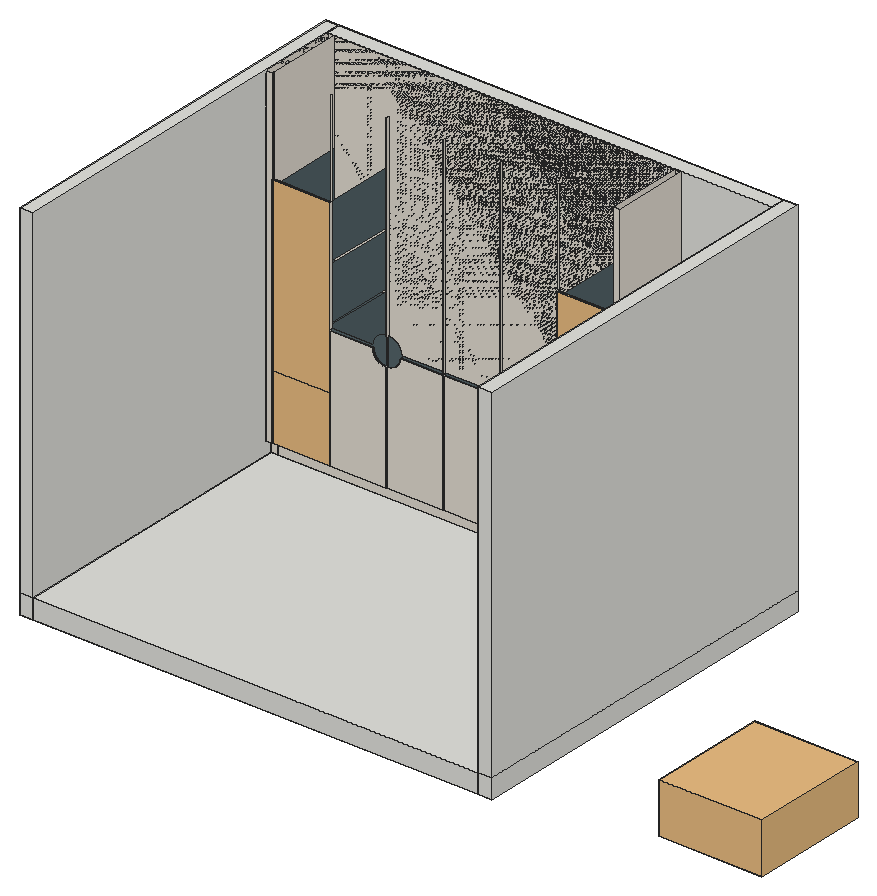
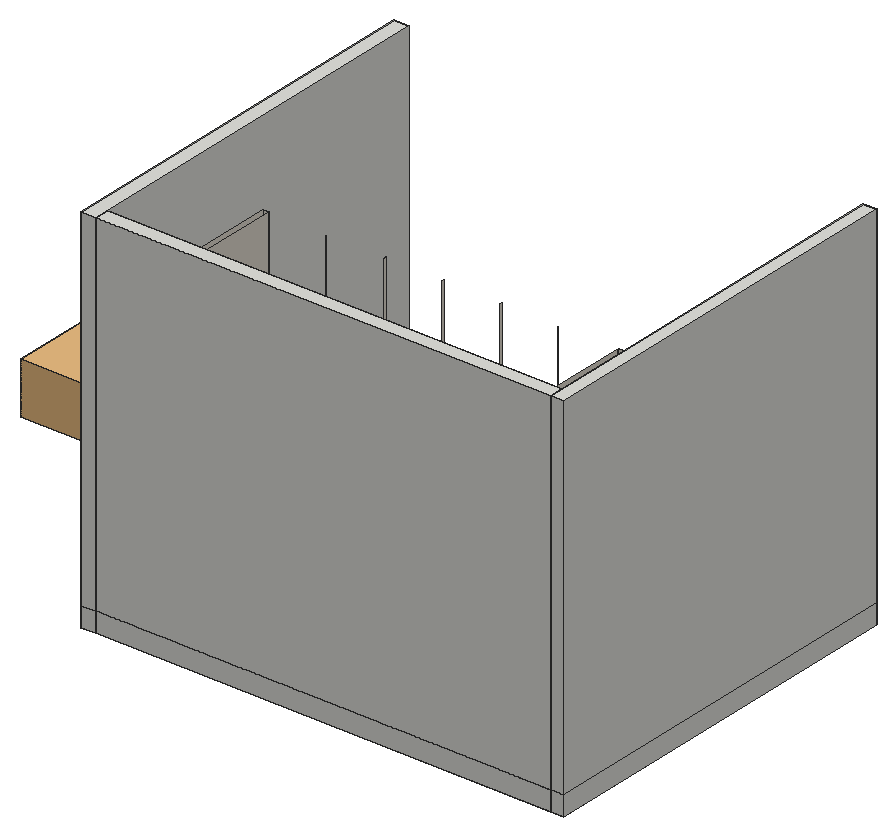
# SketchUp Ruby script. Lengths in millimetres.
U = 1.mm
M = Sketchup.active_model
def pt(a) = Geom::Point3d.new(a.map { |v| v * U })
def face(e, loops, mat)
  f = e.add_face(loops[0].map { |a| pt(a) })
  loops[1..].each { |l| e.add_face(l.map { |a| pt(a) }).erase! }
  f.material = f.back_material = mat if mat
  f
end
# faces: each face lists its corners as indices into pts; further lists are holes
def faces(e, pts, list, mat = nil) = list.each { |f| face(e, (f[0].is_a?(Array) ? f : [f]).map { |l| l.map { |i| pts[i] } }, mat) }
# xy, xz, yz: faces in a plane at the given z, y or x. An outline is a flat list of corners, or four numbers for a rectangle; further outlines are holes
def ring(l) = l.size == 4 ? [[l[0], l[1]], [l[2], l[1]], [l[2], l[3]], [l[0], l[3]]] : l.each_slice(2).to_a
def flat(e, list, mat, &to3) = list.each { |f| face(e, (f[0].is_a?(Array) ? f : [f]).map { |l| ring(l).map { |u, v| to3.(u, v) } }, mat) }
def xy(e, z, list, mat = nil) = flat(e, list, mat) { |x, y| [x, y, z] }
def xz(e, y, list, mat = nil) = flat(e, list, mat) { |x, z| [x, y, z] }
def yz(e, x, list, mat = nil) = flat(e, list, mat) { |y, z| [x, y, z] }
def lines(e, pts, list) = list.each { |a, b| e.add_line(pt(pts[a]), pt(pts[b])) }
# prism: a flat outline (further loops are holes) pulled along v
def prism(e, loops, v, mat = nil)
  f = face(e, loops, mat); d = Geom::Vector3d.new(v.map { |x| x * U })
  f.pushpull(f.normal.samedirection?(d) ? d.length : -d.length)
end
def box(e, o, s, mat = nil) = prism(e, [[o, [o[0] + s[0], o[1], o[2]], [o[0] + s[0], o[1] + s[1], o[2]], [o[0], o[1] + s[1], o[2]]]], [0, 0, s[2]], mat)
def at(x, y, z, deg = 0) = Geom::Transformation.translation(pt([x, y, z])) * Geom::Transformation.rotation(ORIGIN, Z_AXIS, deg.degrees)
def axes(o, x, y, z) = Geom::Transformation.new([*x, 0, *y, 0, *z, 0, *pt(o).to_a, 1])
def part(name) = M.definitions.add(name)
# library, detail: a bought-in or finely detailed component or shape, given as its bounding box
def library(name, o, s) = part(name).tap { |d| box(d.entities, o, s) }
def detail(e, o, s) = box(e.add_group.entities, o, s)
def put(e, d, t, mat = nil) = e.add_instance(d, t).tap { |i| i.material = mat if mat }
def group(e, t, mat = nil) = e.add_group.tap { |g| g.transformation = t; g.material = mat if mat }.entities
root = M.entities
M.materials.add("Olon-Denim-Chic-VT14-1K").color = [84, 100, 105]
M.materials.add("Olon-Fresh-Linen-VT10-1K").color = [226, 220, 209]
M.materials.add("Pionite-a-Panolam-Brand-Tidal-Pool-SB045-4K").color = [68, 97, 103]
c1 = part("Group\#1")
xy(c1.entities,0,[[12.7,0,114.3,3048],[114.3,0,3657.6,3048],[3657.6,0,3771.9,3048]])
xy(c1.entities,152.4,[[12.7,0,114.3,3048],[114.3,0,3657.6,3048],[3657.6,0,3771.9,3048]])
xz(c1.entities,0,[[12.7,0,114.3,152.4],[114.3,0,3657.6,152.4],[3657.6,0,3771.9,152.4]])
xz(c1.entities,3048,[[12.7,0,114.3,152.4],[114.3,0,3657.6,152.4],[3657.6,0,3771.9,152.4]])
yz(c1.entities,12.7,[[0,0,3048,152.4]])
yz(c1.entities,114.3,[[0,0,3048,152.4]])
yz(c1.entities,3657.6,[[0,0,3048,152.4]])
yz(c1.entities,3771.9,[[0,0,3048,152.4]])
xy(root,152.4,[[101.6,2374.9,152.4,2933.7],[152.4,2374.9,2870.2,2933.7],[2870.2,2374.9,2921,2933.7]],"Olon-Fresh-Linen-VT10-1K")
xy(root,254,[[101.6,2324.1,101.6,2374.9,152.4,2374.9,152.4,2342.1,149.4,2342.1,149.4,2324.1],[608.4,2324.1,608.4,2342.1,152.4,2342.1,152.4,2374.9,2870.2,2374.9,2870.2,2342.1,2414.2,2342.1,2414.2,2324.1,1967.3,2324.1,1967.3,2342.1,1964.3,2342.1,1964.3,2324.1,1514.3,2324.1,1514.3,2342.1,1511.3,2342.1,1511.3,2324.1,1061.3,2324.1,1061.3,2342.1,1058.3,2342.1,1058.3,2324.1],[2873.2,2324.1,2873.2,2342.1,2870.2,2342.1,2870.2,2374.9,2921,2374.9,2921,2324.1]],"Olon-Fresh-Linen-VT10-1K")
xy(root,279.4,[[177.8,2342.1,580,2904.1],[2442.6,2342.1,2844.8,2904.1]],"Olon-Denim-Chic-VT14-1K")
xy(root,746.5,[[177.8,2342.1,580,2904.1],[2442.6,2342.1,2844.8,2904.1]],"Olon-Denim-Chic-VT14-1K")
xy(root,797.3,[[177.8,2342.1,580,2904.1]],"Olon-Denim-Chic-VT14-1K")
xy(root,797.3,[[2442.6,2342.1,2844.8,2904.1]],"Pionite-a-Panolam-Brand-Tidal-Pool-SB045-4K")
xy(root,1114.7,[[1054.9,2324.1,1058.3,2333.1],[1061.3,2324.1,1064.8,2333.1],[1960.8,2324.1,1964.3,2333.1],[1967.3,2324.1,1970.7,2333.1]],"Olon-Denim-Chic-VT14-1K")
xy(root,1216.3,[[608.4,2324.1,948.1,2333.1]],"Olon-Denim-Chic-VT14-1K")
xz(root,2324.1,[[101.6,254,149.4,2895.6],[608.4,254,1058.3,254,1058.3,1114.7,1054.9,1114.7,1051.4,1114.9,1047.9,1115.2,1044.5,1115.5,1041,1116,1037.6,1116.6,1034.2,1117.3,1030.8,1118.1,1024.2,1120.1,1020.9,1121.2,1017.6,1122.4,1011.2,1125.2,1008.1,1126.7,1005.1,1128.3,1002,1130.1,999.1,1131.9,996.2,1133.8,993.3,1135.8,990.5,1137.9,987.8,1140,982.6,1144.6,980.1,1147.1,977.7,1149.6,975.4,1152.1,973.1,1154.8,970.9,1157.5,966.9,1163.1,965,1166,963.1,1169,961.4,1172,959.8,1175.1,956.8,1181.3,955.5,1184.5,953.1,1191.1,952.1,1194.4,951.2,1197.8,950.4,1201.1,949.7,1204.5,949.1,1208,948.6,1211.4,948.2,1214.9,948.1,1216.3,608.4,1216.3],[1061.3,254,1511.3,254,1511.3,1216.3,1171.6,1216.3,1171.4,1214.9,1171.1,1211.4,1170.6,1208,1170,1204.5,1169.3,1201.1,1168.5,1197.8,1167.5,1194.4,1166.5,1191.1,1165.4,1187.8,1164.2,1184.5,1162.8,1181.3,1161.4,1178.2,1159.9,1175.1,1158.3,1172,1154.7,1166,1152.8,1163.1,1150.8,1160.3,1148.7,1157.5,1146.6,1154.8,1144.3,1152.1,1142,1149.6,1137,1144.6,1134.5,1142.3,1131.8,1140,1129.1,1137.9,1126.3,1135.8,1123.5,1133.8,1120.6,1131.9,1114.6,1128.3,1111.5,1126.7,1108.4,1125.2,1105.3,1123.8,1102,1122.4,1098.8,1121.2,1095.5,1120.1,1092.2,1119.1,1088.8,1118.1,1085.5,1117.3,1082.1,1116.6,1078.6,1116,1075.2,1115.5,1071.7,1115.2,1068.3,1114.9,1064.8,1114.7,1061.3,1114.7],[1514.3,254,1964.3,254,1964.3,1114.7,1960.8,1114.7,1957.3,1114.9,1953.9,1115.2,1950.4,1115.5,1947,1116,1943.5,1116.6,1940.1,1117.3,1936.8,1118.1,1933.4,1119.1,1930.1,1120.1,1926.8,1121.2,1923.6,1122.4,1920.3,1123.8,1917.2,1125.2,1914.1,1126.7,1911,1128.3,1905,1131.9,1902.1,1133.8,1899.3,1135.8,1896.5,1137.9,1893.8,1140,1891.1,1142.3,1888.6,1144.6,1883.6,1149.6,1881.3,1152.1,1879,1154.8,1876.9,1157.5,1874.8,1160.3,1872.8,1163.1,1870.9,1166,1867.3,1172,1865.7,1175.1,1864.2,1178.2,1862.8,1181.3,1861.4,1184.5,1860.2,1187.8,1859.1,1191.1,1858.1,1194.4,1857.1,1197.8,1856.3,1201.1,1855.6,1204.5,1855,1208,1854.5,1211.4,1854.2,1214.9,1854,1216.3,1514.3,1216.3],[1967.3,254,2414.2,254,2414.2,1216.3,2077.5,1216.3,2077.4,1214.9,2077,1211.4,2076.5,1208,2075.9,1204.5,2075.2,1201.1,2074.4,1197.8,2073.5,1194.4,2072.5,1191.1,2070.1,1184.5,2068.8,1181.3,2065.8,1175.1,2064.2,1172,2062.5,1169,2060.6,1166,2058.7,1163.1,2054.7,1157.5,2052.5,1154.8,2050.2,1152.1,2047.9,1149.6,2045.5,1147.1,2043,1144.6,2037.8,1140,2035.1,1137.9,2032.3,1135.8,2029.4,1133.8,2026.5,1131.9,2023.6,1130.1,2020.5,1128.3,2017.5,1126.7,2014.4,1125.2,2008,1122.4,2004.7,1121.2,2001.4,1120.1,1994.8,1118.1,1991.4,1117.3,1988,1116.6,1984.6,1116,1981.1,1115.5,1977.7,1115.2,1974.2,1114.9,1970.7,1114.7,1967.3,1114.7],
  [2873.2,254,2921,2895.6]],"Olon-Fresh-Linen-VT10-1K")
xz(root,2333.1,[[1054.9,1114.7,1058.3,1114.7,1058.3,1335.9,1054.9,1335.8,1047.9,1335.4,1044.5,1335,1041,1334.5,1037.6,1333.9,1034.2,1333.2,1030.8,1332.4,1027.5,1331.5,1020.9,1329.3,1017.6,1328.1,1014.4,1326.8,1011.2,1325.3,1008.1,1323.8,1005.1,1322.2,1002,1320.5,996.2,1316.7,993.3,1314.7,990.5,1312.7,987.8,1310.5,982.6,1305.9,980.1,1303.5,977.7,1301,973.1,1295.8,970.9,1293.1,968.9,1290.3,966.9,1287.4,963.1,1281.6,961.4,1278.5,959.8,1275.5,958.3,1272.4,956.8,1269.2,955.5,1266,953.1,1259.4,952.1,1256.1,951.2,1252.8,950.4,1249.4,949.7,1246,949.1,1242.6,948.6,1239.1,948.2,1235.7,948.1,1234.3,608.4,1234.3,608.4,1216.3,948.1,1216.3,948.2,1214.9,948.6,1211.4,949.1,1208,949.7,1204.5,950.4,1201.1,951.2,1197.8,952.1,1194.4,953.1,1191.1,955.5,1184.5,956.8,1181.3,959.8,1175.1,961.4,1172,963.1,1169,965,1166,966.9,1163.1,970.9,1157.5,973.1,1154.8,975.4,1152.1,977.7,1149.6,980.1,1147.1,982.6,1144.6,987.8,1140,990.5,1137.9,993.3,1135.8,996.2,1133.8,999.1,1131.9,1002,1130.1,1005.1,1128.3,1008.1,1126.7,1011.2,1125.2,1017.6,1122.4,1020.9,1121.2,1024.2,1120.1,1030.8,1118.1,1034.2,1117.3,1037.6,1116.6,1041,1116,1044.5,1115.5,1047.9,1115.2,1051.4,1114.9],[1061.3,1114.7,1064.8,1114.7,1068.3,1114.9,1071.7,1115.2,1075.2,1115.5,1078.6,1116,1082.1,1116.6,1085.5,1117.3,1088.8,1118.1,1092.2,1119.1,1095.5,1120.1,1098.8,1121.2,1102,1122.4,1105.3,1123.8,1108.4,1125.2,1111.5,1126.7,1114.6,1128.3,1120.6,1131.9,1123.5,1133.8,1126.3,1135.8,1129.1,1137.9,1131.8,1140,1134.5,1142.3,1137,1144.6,1142,1149.6,1144.3,1152.1,1146.6,1154.8,1148.7,1157.5,1150.8,1160.3,1152.8,1163.1,1154.7,1166,1158.3,1172,1159.9,1175.1,1161.4,1178.2,1162.8,1181.3,1164.2,1184.5,1165.4,1187.8,1166.5,1191.1,1167.5,1194.4,1168.5,1197.8,1169.3,1201.1,1170,1204.5,1170.6,1208,1171.1,1211.4,1171.4,1214.9,1171.6,1216.3,1511.3,1216.3,1511.3,1234.3,1171.6,1234.3,1171.4,1235.7,1171.1,1239.1,1170.6,1242.6,1170,1246,1169.3,1249.4,1168.5,1252.8,1166.5,1259.4,1165.4,1262.7,1164.2,1266,1161.4,1272.4,1159.9,1275.5,1158.3,1278.5,1156.5,1281.6,1154.7,1284.5,1152.8,1287.4,1150.8,1290.3,1148.7,1293.1,1146.6,1295.8,1142,1301,1139.5,1303.5,1137,1305.9,1134.5,1308.2,1131.8,1310.5,1129.1,1312.7,1123.5,1316.7,1120.6,1318.6,1117.6,1320.5,1114.6,1322.2,1111.5,1323.8,1105.3,1326.8,1102,1328.1,1098.8,1329.3,1092.2,1331.5,1088.8,1332.4,1085.5,1333.2,1082.1,1333.9,1078.6,1334.5,1075.2,1335,1071.7,1335.4,1068.3,1335.6,1064.8,1335.8,1061.3,1335.9],[1960.8,1114.7,1964.3,1114.7,1964.3,1335.9,1960.8,1335.8,1957.3,1335.6,1953.9,1335.4,1950.4,1335,1947,1334.5,1943.5,1333.9,1940.1,1333.2,1936.8,1332.4,1933.4,1331.5,1926.8,1329.3,1923.6,1328.1,1920.3,1326.8,1914.1,1323.8,1911,1322.2,1908,1320.5,1905,1318.6,1902.1,1316.7,1896.5,1312.7,1893.8,1310.5,1891.1,1308.2,1888.6,1305.9,1886.1,1303.5,1883.6,1301,1879,1295.8,1876.9,1293.1,1874.8,1290.3,1872.8,1287.4,1870.9,1284.5,1869.1,1281.6,1867.3,1278.5,1865.7,1275.5,1864.2,1272.4,1861.4,1266,1860.2,1262.7,1859.1,1259.4,1857.1,1252.8,1856.3,1249.4,1855.6,1246,1855,1242.6,1854.5,1239.1,1854.2,1235.7,1854,1234.3,1514.3,1234.3,1514.3,1216.3,1854,1216.3,1854.2,1214.9,1854.5,1211.4,1855,1208,1855.6,1204.5,1856.3,1201.1,1857.1,1197.8,1858.1,1194.4,1859.1,1191.1,1860.2,1187.8,1861.4,1184.5,1862.8,1181.3,1864.2,1178.2,1865.7,1175.1,1867.3,1172,1870.9,1166,1872.8,1163.1,1874.8,1160.3,1876.9,1157.5,1879,1154.8,1881.3,1152.1,1883.6,1149.6,1888.6,1144.6,1891.1,1142.3,1893.8,1140,1896.5,1137.9,1899.3,1135.8,1902.1,1133.8,1905,1131.9,1911,1128.3,1914.1,1126.7,1917.2,1125.2,1920.3,1123.8,1923.6,1122.4,1926.8,1121.2,1930.1,1120.1,1933.4,1119.1,1936.8,1118.1,1940.1,1117.3,1943.5,1116.6,1947,1116,1950.4,1115.5,1953.9,1115.2,1957.3,1114.9],[1967.3,1114.7,1970.7,1114.7,1974.2,1114.9,1977.7,1115.2,1981.1,1115.5,1984.6,1116,1988,1116.6,1991.4,1117.3,1994.8,1118.1,2001.4,1120.1,2004.7,1121.2,2008,1122.4,2014.4,1125.2,2017.5,1126.7,2020.5,1128.3,2023.6,1130.1,2026.5,1131.9,2029.4,1133.8,2032.3,1135.8,2035.1,1137.9,2037.8,1140,2043,1144.6,2045.5,1147.1,2047.9,1149.6,2050.2,1152.1,2052.5,1154.8,2054.7,1157.5,2058.7,1163.1,2060.6,1166,2062.5,1169,2064.2,1172,2065.8,1175.1,2068.8,1181.3,2070.1,1184.5,2072.5,1191.1,2073.5,1194.4,2074.4,1197.8,2075.2,1201.1,2075.9,1204.5,2076.5,1208,2077,1211.4,2077.4,1214.9,2077.5,1216.3,2414.2,1216.3,2414.2,1234.3,2077.5,1234.3,2077.4,1235.7,2077,1239.1,2076.5,1242.6,2075.9,1246,2075.2,1249.4,2074.4,1252.8,2073.5,1256.1,2072.5,1259.4,2070.1,1266,2068.8,1269.2,2067.3,1272.4,2065.8,1275.5,2064.2,1278.5,2062.5,1281.6,2058.7,1287.4,2056.7,1290.3,2054.7,1293.1,2052.5,1295.8,2047.9,1301,2045.5,1303.5,2043,1305.9,2037.8,1310.5,2035.1,1312.7,2032.3,1314.7,2029.4,1316.7,2023.6,1320.5,2020.5,1322.2,2017.5,1323.8,2014.4,1325.3,2011.2,1326.8,2008,1328.1,2004.7,1329.3,1998.1,1331.5,1994.8,1332.4,1991.4,1333.2,1988,1333.9,1984.6,1334.5,1981.1,1335,1977.7,1335.4,1970.7,1335.8,1967.3,1335.9]],"Olon-Denim-Chic-VT14-1K")
xz(root,2342.1,[[149.4,254,152.4,2895.6],[[152.4,254,605.4,770.4],[177.8,279.4,580,746.5]],[605.4,254,608.4,2895.6],[1058.3,254,1061.3,2895.6],[1511.3,254,1514.3,2895.6],
  [1964.3,254,1967.3,2895.6],[2414.2,254,2417.2,2895.6],[[2417.2,254,2870.2,770.4],[2442.6,279.4,2844.8,746.5]],[2870.2,254,2873.2,2895.6],[152.4,770.4,605.4,773.4],
  [2417.2,770.4,2870.2,773.4],[[152.4,773.4,605.4,2132.1],[177.8,797.3,580,2108.2]],[[2417.2,773.4,2870.2,2132.1],[2442.6,797.3,2844.8,2108.2]]],"Olon-Fresh-Linen-VT10-1K")
xz(root,2374.9,[[101.6,152.4,152.4,254],[152.4,152.4,2870.2,254],[2870.2,152.4,2921,254]],"Olon-Fresh-Linen-VT10-1K")
xz(root,2904.1,[[177.8,279.4,580,746.5],[2442.6,279.4,2844.8,746.5],[177.8,797.3,580,1225.3],[2442.6,797.3,2844.8,1225.3]],"Olon-Denim-Chic-VT14-1K")
xz(root,2933.7,[[101.6,152.4,152.4,2895.6],[152.4,152.4,2870.2,2895.6],[2870.2,152.4,2921,2895.6]],"Olon-Fresh-Linen-VT10-1K")
yz(root,101.6,[[2374.9,152.4,2374.9,254,2324.1,254,2324.1,2895.6,2933.7,2895.6,2933.7,152.4]],"Olon-Fresh-Linen-VT10-1K")
yz(root,149.4,[[2324.1,254,2342.1,770.4],[2324.1,770.4,2342.1,773.4],[2324.1,773.4,2342.1,2132.1]],"Olon-Fresh-Linen-VT10-1K")
yz(root,152.4,[[2374.9,152.4,2933.7,152.4,2933.7,2895.6,2342.1,2895.6,2342.1,254,2374.9,254]],"Olon-Fresh-Linen-VT10-1K")
yz(root,177.8,[[2342.1,279.4,2904.1,746.5],[2342.1,797.3,2904.1,797.3,2904.1,1225.3,2344.1,1225.3,2344.1,1243.3,2904.1,1243.3,2904.1,1662.2,2344.1,1662.2,2344.1,1680.2,2904.1,1680.2,2904.1,2108.2,2342.1,2108.2]],"Olon-Denim-Chic-VT14-1K")
yz(root,580,[[2342.1,279.4,2904.1,746.5],[2342.1,797.3,2342.1,2108.2,2904.1,2108.2,2904.1,1680.2,2344.1,1680.2,2344.1,1662.2,2904.1,1662.2,2904.1,1243.3,2344.1,1243.3,2344.1,1225.3,2904.1,1225.3,2904.1,797.3]],"Olon-Denim-Chic-VT14-1K")
yz(root,608.4,[[2324.1,254,2342.1,770.4],[2324.1,770.4,2342.1,773.4],[2324.1,773.4,2324.1,1216.3,2333.1,1216.3,2333.1,1234.3,2324.1,1234.3,2324.1,2132.1,2342.1,2132.1,2342.1,773.4]],"Olon-Fresh-Linen-VT10-1K")
yz(root,1058.3,[[2324.1,254,2342.1,254,2342.1,2895.6,2324.1,2895.6,2324.1,1335.9,2333.1,1335.9,2333.1,1114.7,2324.1,1114.7]],"Olon-Fresh-Linen-VT10-1K")
yz(root,1061.3,[[2324.1,254,2324.1,1114.7,2333.1,1114.7,2333.1,1335.9,2324.1,1335.9,2324.1,2895.6,2342.1,2895.6,2342.1,254]],"Olon-Fresh-Linen-VT10-1K")
yz(root,1511.3,[[2324.1,254,2342.1,254,2342.1,2895.6,2324.1,2895.6,2324.1,1234.3,2333.1,1234.3,2333.1,1216.3,2324.1,1216.3]],"Olon-Fresh-Linen-VT10-1K")
yz(root,1514.3,[[2324.1,254,2324.1,1216.3,2333.1,1216.3,2333.1,1234.3,2324.1,1234.3,2324.1,2895.6,2342.1,2895.6,2342.1,254]],"Olon-Fresh-Linen-VT10-1K")
yz(root,1964.3,[[2324.1,254,2342.1,254,2342.1,2895.6,2324.1,2895.6,2324.1,1335.9,2333.1,1335.9,2333.1,1114.7,2324.1,1114.7]],"Olon-Fresh-Linen-VT10-1K")
yz(root,1967.3,[[2324.1,254,2324.1,1114.7,2333.1,1114.7,2333.1,1335.9,2324.1,1335.9,2324.1,2895.6,2342.1,2895.6,2342.1,254]],"Olon-Fresh-Linen-VT10-1K")
yz(root,2414.2,[[2324.1,254,2342.1,771.9],[2324.1,771.9,2342.1,771.9,2342.1,2133.6,2324.1,2133.6,2324.1,1234.3,2333.1,1234.3,2333.1,1216.3,2324.1,1216.3]],"Olon-Fresh-Linen-VT10-1K")
yz(root,2442.6,[[2342.1,279.4,2904.1,746.5],[2342.1,797.3,2904.1,797.3,2904.1,1225.3,2362.1,1225.3,2362.1,1243.3,2904.1,1243.3,2904.1,1662.2,2362.1,1662.2,2362.1,1680.2,2904.1,1680.2,2904.1,2108.2,2342.1,2108.2]],"Olon-Denim-Chic-VT14-1K")
yz(root,2844.8,[[2342.1,279.4,2904.1,746.5],[2342.1,797.3,2904.1,1225.3]],"Olon-Denim-Chic-VT14-1K")
yz(root,2870.2,[[2374.9,152.4,2374.9,254,2342.1,254,2342.1,2895.6,2933.7,2895.6,2933.7,152.4]],"Olon-Fresh-Linen-VT10-1K")
yz(root,2873.2,[[2324.1,254,2342.1,771.9],[2324.1,771.9,2342.1,2133.6]],"Olon-Fresh-Linen-VT10-1K")
yz(root,2921,[[2374.9,152.4,2933.7,152.4,2933.7,2895.6,2324.1,2895.6,2324.1,254,2374.9,254]],"Olon-Fresh-Linen-VT10-1K")
p = [[1051.4,2324.1,1114.9],[1054.9,2324.1,1114.7],[1054.9,2333.1,1114.7],[1051.4,2333.1,1114.9],[1064.8,2324.1,1114.7],[1068.3,2324.1,1114.9],
  [1068.3,2333.1,1114.9],[1064.8,2333.1,1114.7],[1957.3,2324.1,1114.9],[1960.8,2324.1,1114.7],[1960.8,2333.1,1114.7],[1957.3,2333.1,1114.9],
  [1970.7,2324.1,1114.7],[1974.2,2324.1,1114.9],[1974.2,2333.1,1114.9],[1970.7,2333.1,1114.7],[1047.9,2324.1,1115.2],[1047.9,2333.1,1115.2],
  [1071.7,2324.1,1115.2],[1071.7,2333.1,1115.2],[1953.9,2324.1,1115.2],[1953.9,2333.1,1115.2],[1977.7,2324.1,1115.2],[1977.7,2333.1,1115.2],
  [1044.5,2324.1,1115.5],[1044.5,2333.1,1115.5],[1075.2,2324.1,1115.5],[1075.2,2333.1,1115.5],[1950.4,2324.1,1115.5],[1950.4,2333.1,1115.5],
  [1981.1,2324.1,1115.5],[1981.1,2333.1,1115.5],[1041,2324.1,1116],[1041,2333.1,1116],[1078.6,2324.1,1116],[1078.6,2333.1,1116],
  [1947,2324.1,1116],[1947,2333.1,1116],[1984.6,2324.1,1116],[1984.6,2333.1,1116],[1037.6,2324.1,1116.6],[1037.6,2333.1,1116.6],
  [1082.1,2324.1,1116.6],[1082.1,2333.1,1116.6],[1943.5,2324.1,1116.6],[1943.5,2333.1,1116.6],[1988,2324.1,1116.6],[1988,2333.1,1116.6],
  [1034.2,2324.1,1117.3],[1034.2,2333.1,1117.3],[1085.5,2324.1,1117.3],[1085.5,2333.1,1117.3],[1940.1,2324.1,1117.3],[1940.1,2333.1,1117.3],
  [1991.4,2324.1,1117.3],[1991.4,2333.1,1117.3],[1030.8,2324.1,1118.1],[1030.8,2333.1,1118.1],[1088.8,2324.1,1118.1],[1088.8,2333.1,1118.1],
  [1936.8,2324.1,1118.1],[1936.8,2333.1,1118.1],[1994.8,2324.1,1118.1],[1994.8,2333.1,1118.1],[1027.5,2324.1,1119.1],[1027.5,2333.1,1119.1],
  [1092.2,2324.1,1119.1],[1092.2,2333.1,1119.1],[1933.4,2324.1,1119.1],[1933.4,2333.1,1119.1],[1998.1,2324.1,1119.1],[1998.1,2333.1,1119.1],
  [1024.2,2324.1,1120.1],[1024.2,2333.1,1120.1],[1095.5,2324.1,1120.1],[1095.5,2333.1,1120.1],[1930.1,2324.1,1120.1],[1930.1,2333.1,1120.1],
  [2001.4,2324.1,1120.1],[2001.4,2333.1,1120.1],[1020.9,2324.1,1121.2],[1020.9,2333.1,1121.2],[1098.8,2324.1,1121.2],[1098.8,2333.1,1121.2],
  [1926.8,2324.1,1121.2],[1926.8,2333.1,1121.2],[2004.7,2324.1,1121.2],[2004.7,2333.1,1121.2],[1017.6,2324.1,1122.4],[1017.6,2333.1,1122.4],
  [1102,2324.1,1122.4],[1102,2333.1,1122.4],[1923.6,2324.1,1122.4],[1923.6,2333.1,1122.4],[2008,2324.1,1122.4],[2008,2333.1,1122.4],
  [1014.4,2324.1,1123.8],[1014.4,2333.1,1123.8],[1105.3,2324.1,1123.8],[1105.3,2333.1,1123.8],[1920.3,2324.1,1123.8],[1920.3,2333.1,1123.8],
  [2011.2,2324.1,1123.8],[2011.2,2333.1,1123.8],[1011.2,2324.1,1125.2],[1011.2,2333.1,1125.2],[1108.4,2324.1,1125.2],[1108.4,2333.1,1125.2],
  [1917.2,2324.1,1125.2],[1917.2,2333.1,1125.2],[2014.4,2324.1,1125.2],[2014.4,2333.1,1125.2],[1008.1,2324.1,1126.7],[1008.1,2333.1,1126.7],
  [1111.5,2324.1,1126.7],[1111.5,2333.1,1126.7],[1914.1,2324.1,1126.7],[1914.1,2333.1,1126.7],[2017.5,2324.1,1126.7],[2017.5,2333.1,1126.7],
  [1005.1,2324.1,1128.3],[1005.1,2333.1,1128.3],[1114.6,2324.1,1128.3],[1114.6,2333.1,1128.3],[1911,2324.1,1128.3],[1911,2333.1,1128.3],
  [2020.5,2324.1,1128.3],[2020.5,2333.1,1128.3],[1002,2324.1,1130.1],[1002,2333.1,1130.1],[1117.6,2324.1,1130.1],[1117.6,2333.1,1130.1],
  [1908,2324.1,1130.1],[1908,2333.1,1130.1],[2023.6,2324.1,1130.1],[2023.6,2333.1,1130.1],[999.1,2324.1,1131.9],[999.1,2333.1,1131.9],
  [1120.6,2324.1,1131.9],[1120.6,2333.1,1131.9],[1905,2324.1,1131.9],[1905,2333.1,1131.9],[2026.5,2324.1,1131.9],[2026.5,2333.1,1131.9],
  [996.2,2324.1,1133.8],[996.2,2333.1,1133.8],[1123.5,2324.1,1133.8],[1123.5,2333.1,1133.8],[1902.1,2324.1,1133.8],[1902.1,2333.1,1133.8],
  [2029.4,2324.1,1133.8],[2029.4,2333.1,1133.8],[993.3,2324.1,1135.8],[993.3,2333.1,1135.8],[1126.3,2324.1,1135.8],[1126.3,2333.1,1135.8],
  [1899.3,2324.1,1135.8],[1899.3,2333.1,1135.8],[2032.3,2324.1,1135.8],[2032.3,2333.1,1135.8],[990.5,2324.1,1137.9],[990.5,2333.1,1137.9],
  [1129.1,2324.1,1137.9],[1129.1,2333.1,1137.9],[1896.5,2324.1,1137.9],[1896.5,2333.1,1137.9],[2035.1,2324.1,1137.9],[2035.1,2333.1,1137.9],
  [987.8,2324.1,1140],[987.8,2333.1,1140],[1131.8,2324.1,1140],[1131.8,2333.1,1140],[1893.8,2324.1,1140],[1893.8,2333.1,1140],
  [2037.8,2324.1,1140],[2037.8,2333.1,1140],[985.2,2324.1,1142.3],[985.2,2333.1,1142.3],[1134.5,2324.1,1142.3],[1134.5,2333.1,1142.3],
  [1891.1,2324.1,1142.3],[1891.1,2333.1,1142.3],[2040.4,2324.1,1142.3],[2040.4,2333.1,1142.3],[982.6,2324.1,1144.6],[982.6,2333.1,1144.6],
  [1137,2324.1,1144.6],[1137,2333.1,1144.6],[1888.6,2324.1,1144.6],[1888.6,2333.1,1144.6],[2043,2324.1,1144.6],[2043,2333.1,1144.6],
  [980.1,2324.1,1147.1],[980.1,2333.1,1147.1],[1139.5,2324.1,1147.1],[1139.5,2333.1,1147.1],[1886.1,2324.1,1147.1],[1886.1,2333.1,1147.1],
  [2045.5,2324.1,1147.1],[2045.5,2333.1,1147.1],[977.7,2324.1,1149.6],[977.7,2333.1,1149.6],[1142,2324.1,1149.6],[1142,2333.1,1149.6],
  [1883.6,2324.1,1149.6],[1883.6,2333.1,1149.6],[2047.9,2324.1,1149.6],[2047.9,2333.1,1149.6],[975.4,2324.1,1152.1],[975.4,2333.1,1152.1],
  [1144.3,2324.1,1152.1],[1144.3,2333.1,1152.1],[1881.3,2324.1,1152.1],[1881.3,2333.1,1152.1],[2050.2,2324.1,1152.1],[2050.2,2333.1,1152.1],
  [973.1,2324.1,1154.8],[973.1,2333.1,1154.8],[1146.6,2324.1,1154.8],[1146.6,2333.1,1154.8],[1879,2324.1,1154.8],[1879,2333.1,1154.8],
  [2052.5,2324.1,1154.8],[2052.5,2333.1,1154.8],[970.9,2324.1,1157.5],[970.9,2333.1,1157.5],[1148.7,2324.1,1157.5],[1148.7,2333.1,1157.5],
  [1876.9,2324.1,1157.5],[1876.9,2333.1,1157.5],[2054.7,2324.1,1157.5],[2054.7,2333.1,1157.5],[968.9,2324.1,1160.3],[968.9,2333.1,1160.3],
  [1150.8,2324.1,1160.3],[1150.8,2333.1,1160.3],[1874.8,2324.1,1160.3],[1874.8,2333.1,1160.3],[2056.7,2324.1,1160.3],[2056.7,2333.1,1160.3],
  [966.9,2324.1,1163.1],[966.9,2333.1,1163.1],[1152.8,2324.1,1163.1],[1152.8,2333.1,1163.1],[1872.8,2324.1,1163.1],[1872.8,2333.1,1163.1],
  [2058.7,2324.1,1163.1],[2058.7,2333.1,1163.1],[965,2324.1,1166],[965,2333.1,1166],[1154.7,2324.1,1166],[1154.7,2333.1,1166],
  [1870.9,2324.1,1166],[1870.9,2333.1,1166],[2060.6,2324.1,1166],[2060.6,2333.1,1166],[963.1,2324.1,1169],[963.1,2333.1,1169],
  [1156.5,2324.1,1169],[1156.5,2333.1,1169],[1869.1,2324.1,1169],[1869.1,2333.1,1169],[2062.5,2324.1,1169],[2062.5,2333.1,1169],
  [961.4,2324.1,1172],[961.4,2333.1,1172],[1158.3,2324.1,1172],[1158.3,2333.1,1172],[1867.3,2324.1,1172],[1867.3,2333.1,1172],
  [2064.2,2324.1,1172],[2064.2,2333.1,1172],[959.8,2324.1,1175.1],[959.8,2333.1,1175.1],[1159.9,2324.1,1175.1],[1159.9,2333.1,1175.1],
  [1865.7,2324.1,1175.1],[1865.7,2333.1,1175.1],[2065.8,2324.1,1175.1],[2065.8,2333.1,1175.1],[958.3,2324.1,1178.2],[958.3,2333.1,1178.2],
  [1161.4,2324.1,1178.2],[1161.4,2333.1,1178.2],[1864.2,2324.1,1178.2],[1864.2,2333.1,1178.2],[2067.3,2324.1,1178.2],[2067.3,2333.1,1178.2],
  [956.8,2324.1,1181.3],[956.8,2333.1,1181.3],[1162.8,2324.1,1181.3],[1162.8,2333.1,1181.3],[1862.8,2324.1,1181.3],[1862.8,2333.1,1181.3],
  [2068.8,2324.1,1181.3],[2068.8,2333.1,1181.3],[955.5,2324.1,1184.5],[955.5,2333.1,1184.5],[1164.2,2324.1,1184.5],[1164.2,2333.1,1184.5],
  [1861.4,2324.1,1184.5],[1861.4,2333.1,1184.5],[2070.1,2324.1,1184.5],[2070.1,2333.1,1184.5],[954.3,2324.1,1187.8],[954.3,2333.1,1187.8],
  [1165.4,2324.1,1187.8],[1165.4,2333.1,1187.8],[1860.2,2324.1,1187.8],[1860.2,2333.1,1187.8],[2071.3,2324.1,1187.8],[2071.3,2333.1,1187.8],
  [953.1,2324.1,1191.1],[953.1,2333.1,1191.1],[1166.5,2324.1,1191.1],[1166.5,2333.1,1191.1],[1859.1,2324.1,1191.1],[1859.1,2333.1,1191.1],
  [2072.5,2324.1,1191.1],[2072.5,2333.1,1191.1],[952.1,2324.1,1194.4],[952.1,2333.1,1194.4],[1167.5,2324.1,1194.4],[1167.5,2333.1,1194.4],
  [1858.1,2324.1,1194.4],[1858.1,2333.1,1194.4],[2073.5,2324.1,1194.4],[2073.5,2333.1,1194.4],[951.2,2324.1,1197.8],[951.2,2333.1,1197.8],
  [1168.5,2324.1,1197.8],[1168.5,2333.1,1197.8],[1857.1,2324.1,1197.8],[1857.1,2333.1,1197.8],[2074.4,2324.1,1197.8],[2074.4,2333.1,1197.8],
  [950.4,2324.1,1201.1],[950.4,2333.1,1201.1],[1169.3,2324.1,1201.1],[1169.3,2333.1,1201.1],[1856.3,2324.1,1201.1],[1856.3,2333.1,1201.1],
  [2075.2,2324.1,1201.1],[2075.2,2333.1,1201.1],[949.7,2324.1,1204.5],[949.7,2333.1,1204.5],[1170,2324.1,1204.5],[1170,2333.1,1204.5],
  [1855.6,2324.1,1204.5],[1855.6,2333.1,1204.5],[2075.9,2324.1,1204.5],[2075.9,2333.1,1204.5],[949.1,2324.1,1208],[949.1,2333.1,1208],
  [1170.6,2324.1,1208],[1170.6,2333.1,1208],[1855,2324.1,1208],[1855,2333.1,1208],[2076.5,2324.1,1208],[2076.5,2333.1,1208],
  [948.6,2324.1,1211.4],[948.6,2333.1,1211.4],[1171.1,2324.1,1211.4],[1171.1,2333.1,1211.4],[1854.5,2324.1,1211.4],[1854.5,2333.1,1211.4],
  [2077,2324.1,1211.4],[2077,2333.1,1211.4],[948.2,2324.1,1214.9],[948.2,2333.1,1214.9],[1171.4,2324.1,1214.9],[1171.4,2333.1,1214.9],
  [1854.2,2324.1,1214.9],[1854.2,2333.1,1214.9],[2077.4,2324.1,1214.9],[2077.4,2333.1,1214.9],[948.1,2324.1,1216.3],[948.1,2333.1,1216.3],
  [1171.6,2324.1,1216.3],[1171.6,2333.1,1216.3],[1854,2324.1,1216.3],[1854,2333.1,1216.3],[2077.5,2324.1,1216.3],[2077.5,2333.1,1216.3],
  [5063.1,641.6,-5.8],[5271.9,521,-5.8],[5480.7,641.6,-5.8],[5063.1,882.7,-5.8],[5480.7,882.7,-5.8],[5271.9,1003.2,-5.8],
  [5063.1,641.6,-17.8],[5271.9,521,-17.8],[5480.7,641.6,-17.8],[5063.1,882.7,-17.8],[5480.7,882.7,-17.8],[5271.9,1003.2,-17.8],
  [5063.1,641.6,-29.8],[5271.9,521,-29.8],[5480.7,641.6,-29.8],[5063.1,882.7,-29.8],[5480.7,882.7,-29.8],[5271.9,1003.2,-29.8],
  [5063.1,641.6,-41.8],[5271.9,521,-41.8],[5480.7,641.6,-41.8],[5063.1,882.7,-41.8],[5480.7,882.7,-41.8],[5271.9,1003.2,-41.8],
  [5063.1,641.6,-53.8],[5271.9,521,-53.8],[5480.7,641.6,-53.8],[5063.1,882.7,-53.8],[5480.7,882.7,-53.8],[5271.9,1003.2,-53.8],
  [5063.1,641.6,-65.8],[5271.9,521,-65.8],[5480.7,641.6,-65.8],[5063.1,882.7,-65.8],[5480.7,882.7,-65.8],[5271.9,1003.2,-65.8],
  [5063.1,641.6,-77.8],[5271.9,521,-77.8],[5480.7,641.6,-77.8],[5063.1,882.7,-77.8],[5480.7,882.7,-77.8],[5271.9,1003.2,-77.8]]
faces(root,p,[[0,1,2,3],[4,5,6,7],[8,9,10,11],[12,13,14,15],[16,0,3,17],[5,18,19,6],[20,8,11,21],[13,22,23,14],
  [24,16,17,25],[18,26,27,19],[28,20,21,29],[22,30,31,23],[32,24,25,33],[26,34,35,27],[36,28,29,37],[30,38,39,31],
  [40,32,33,41],[34,42,43,35],[44,36,37,45],[38,46,47,39],[48,40,41,49],[42,50,51,43],[52,44,45,53],[46,54,55,47],
  [56,48,49,57],[50,58,59,51],[60,52,53,61],[54,62,63,55],[64,56,57,65],[58,66,67,59],[68,60,61,69],[62,70,71,63],
  [72,64,65,73],[66,74,75,67],[76,68,69,77],[70,78,79,71],[80,72,73,81],[74,82,83,75],[84,76,77,85],[78,86,87,79],
  [88,80,81,89],[82,90,91,83],[92,84,85,93],[86,94,95,87],[96,88,89,97],[90,98,99,91],[100,92,93,101],[94,102,103,95],
  [104,96,97,105],[98,106,107,99],[108,100,101,109],[102,110,111,103],[112,104,105,113],[106,114,115,107],[116,108,109,117],[110,118,119,111],
  [120,112,113,121],[114,122,123,115],[124,116,117,125],[118,126,127,119],[128,120,121,129],[122,130,131,123],[132,124,125,133],[126,134,135,127],
  [136,128,129,137],[130,138,139,131],[140,132,133,141],[134,142,143,135],[144,136,137,145],[138,146,147,139],[148,140,141,149],[142,150,151,143],
  [152,144,145,153],[146,154,155,147],[156,148,149,157],[150,158,159,151],[160,152,153,161],[154,162,163,155],[164,156,157,165],[158,166,167,159],
  [168,160,161,169],[162,170,171,163],[172,164,165,173],[166,174,175,167],[176,168,169,177],[170,178,179,171],[180,172,173,181],[174,182,183,175],
  [184,176,177,185],[178,186,187,179],[188,180,181,189],[182,190,191,183],[192,184,185,193],[186,194,195,187],[196,188,189,197],[190,198,199,191],
  [200,192,193,201],[194,202,203,195],[204,196,197,205],[198,206,207,199],[208,200,201,209],[202,210,211,203],[212,204,205,213],[206,214,215,207],
  [216,208,209,217],[210,218,219,211],[220,212,213,221],[214,222,223,215],[224,216,217,225],[218,226,227,219],[228,220,221,229],[222,230,231,223],
  [232,224,225,233],[226,234,235,227],[236,228,229,237],[230,238,239,231],[240,232,233,241],[234,242,243,235],[244,236,237,245],[238,246,247,239],
  [248,240,241,249],[242,250,251,243],[252,244,245,253],[246,254,255,247],[256,248,249,257],[250,258,259,251],[260,252,253,261],[254,262,263,255],
  [264,256,257,265],[258,266,267,259],[268,260,261,269],[262,270,271,263],[272,264,265,273],[266,274,275,267],[276,268,269,277],[270,278,279,271],
  [280,272,273,281],[274,282,283,275],[284,276,277,285],[278,286,287,279],[288,280,281,289],[282,290,291,283],[292,284,285,293],[286,294,295,287],
  [296,288,289,297],[290,298,299,291],[300,292,293,301],[294,302,303,295],[304,296,297,305],[298,306,307,299],[308,300,301,309],[302,310,311,303],
  [312,304,305,313],[306,314,315,307],[316,308,309,317],[310,318,319,311],[320,312,313,321],[314,322,323,315],[324,316,317,325],[318,326,327,319],
  [328,320,321,329],[322,330,331,323],[332,324,325,333],[326,334,335,327],[336,328,329,337],[330,338,339,331],[340,332,333,341],[334,342,343,335],
  [344,336,337,345],[338,346,347,339],[348,340,341,349],[342,350,351,343],[352,344,345,353],[346,354,355,347],[356,348,349,357],[350,358,359,351],
  [360,352,353,361],[354,362,363,355],[364,356,357,365],[358,366,367,359],[368,360,361,369],[362,370,371,363],[372,364,365,373],[366,374,375,367],
  [376,368,369,377],[370,378,379,371],[380,372,373,381],[374,382,383,375]],"Olon-Denim-Chic-VT14-1K")
lines(root,p,[[384,385],[385,386],[387,384],[386,388],[389,388],[387,389],[390,391],[391,392],[393,390],[392,394],[395,394],[393,395],
  [396,397],[397,398],[399,396],[398,400],[401,400],[399,401],[402,403],[403,404],[405,402],[404,406],[407,406],[405,407],
  [408,409],[409,410],[411,408],[410,412],[413,412],[411,413],[414,415],[415,416],[417,414],[416,418],[419,418],[417,419],
  [420,421],[421,422],[423,420],[422,424],[425,424],[423,425]])
detail(root,[4860.8,287.5,0],[822.2,949.3,401.6])
put(root,c1,at(-12.7,0,0))
g1 = group(root,at(-12.7,2933.7,152.4))
box(g1,[114.3,0,0],[3543.3,114.3,2749.2])
g2 = group(root,at(0,0,152.4))
box(g2,[0,0,0],[101.6,3048,2749.2])
g3 = group(root,at(3644.9,0,152.4))
box(g3,[0,0,0],[114.3,3048,2749.2])
g4 = group(root,at(152.4,2324.1,254),"Olon-Fresh-Linen-VT10-1K")
detail(g4,[0,0,0],[453,18,516.4])
g5 = group(root,at(2417.2,2324.1,254),"Olon-Fresh-Linen-VT10-1K")
detail(g5,[0,0,0],[453,18,516.4])
g6 = group(root,at(152.4,2324.1,773.4),"Olon-Fresh-Linen-VT10-1K")
detail(g6,[0,0,0],[453,18,1358.7])
g7 = group(root,at(2417.2,2324.1,773.4),"Olon-Fresh-Linen-VT10-1K")
detail(g7,[0,0,0],[453,18,1358.7])
